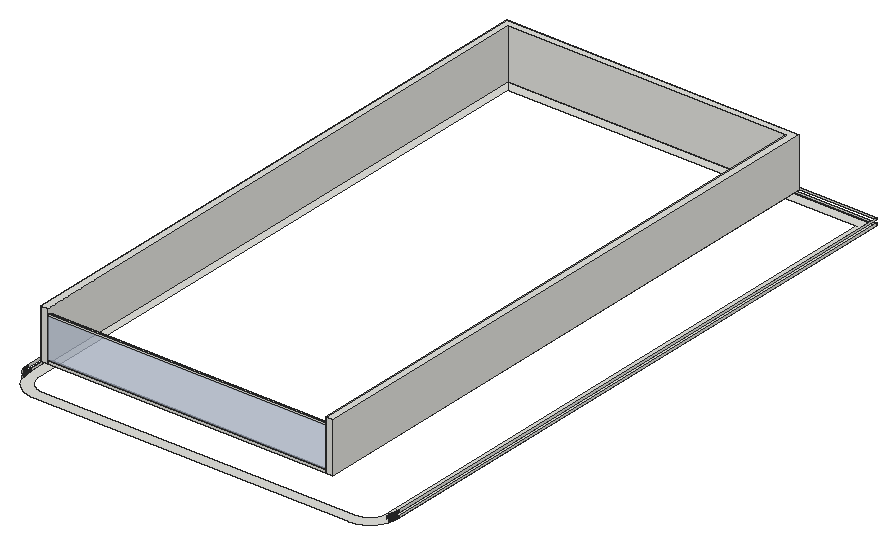
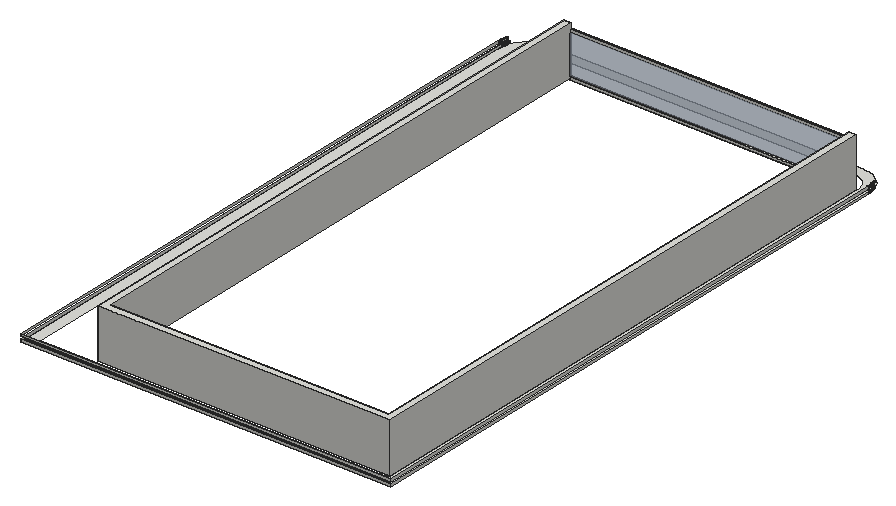
# SketchUp Ruby script. Lengths in inches.
U = 1.inch
M = Sketchup.active_model
def pt(a) = Geom::Point3d.new(a.map { |v| v * U })
def face(e, loops, mat)
  f = e.add_face(loops[0].map { |a| pt(a) })
  loops[1..].each { |l| e.add_face(l.map { |a| pt(a) }).erase! }
  f.material = f.back_material = mat if mat
  f
end
# faces: each face lists its corners as indices into pts; further lists are holes
def faces(e, pts, list, mat = nil) = list.each { |f| face(e, (f[0].is_a?(Array) ? f : [f]).map { |l| l.map { |i| pts[i] } }, mat) }
# xy, xz, yz: faces in a plane at the given z, y or x. An outline is a flat list of corners, or four numbers for a rectangle; further outlines are holes
def ring(l) = l.size == 4 ? [[l[0], l[1]], [l[2], l[1]], [l[2], l[3]], [l[0], l[3]]] : l.each_slice(2).to_a
def flat(e, list, mat, &to3) = list.each { |f| face(e, (f[0].is_a?(Array) ? f : [f]).map { |l| ring(l).map { |u, v| to3.(u, v) } }, mat) }
def xy(e, z, list, mat = nil) = flat(e, list, mat) { |x, y| [x, y, z] }
def xz(e, y, list, mat = nil) = flat(e, list, mat) { |x, z| [x, y, z] }
def yz(e, x, list, mat = nil) = flat(e, list, mat) { |y, z| [x, y, z] }
def lines(e, pts, list) = list.each { |a, b| e.add_line(pt(pts[a]), pt(pts[b])) }
# prism: a flat outline (further loops are holes) pulled along v
def prism(e, loops, v, mat = nil)
  f = face(e, loops, mat); d = Geom::Vector3d.new(v.map { |x| x * U })
  f.pushpull(f.normal.samedirection?(d) ? d.length : -d.length)
end
def box(e, o, s, mat = nil) = prism(e, [[o, [o[0] + s[0], o[1], o[2]], [o[0] + s[0], o[1] + s[1], o[2]], [o[0], o[1] + s[1], o[2]]]], [0, 0, s[2]], mat)
def at(x, y, z, deg = 0) = Geom::Transformation.translation(pt([x, y, z])) * Geom::Transformation.rotation(ORIGIN, Z_AXIS, deg.degrees)
def axes(o, x, y, z) = Geom::Transformation.new([*x, 0, *y, 0, *z, 0, *pt(o).to_a, 1])
def part(name) = M.definitions.add(name)
# library, detail: a bought-in or finely detailed component or shape, given as its bounding box
def library(name, o, s) = part(name).tap { |d| box(d.entities, o, s) }
def detail(e, o, s) = box(e.add_group.entities, o, s)
def put(e, d, t, mat = nil) = e.add_instance(d, t).tap { |i| i.material = mat if mat }
def group(e, t, mat = nil) = e.add_group.tap { |g| g.transformation = t; g.material = mat if mat }.entities
root = M.entities
M.materials.add("[Translucent Glass Blue]").color = [196, 207, 226]
M.materials["[Translucent Glass Blue]"].alpha = 0.5
xy(root,392.81,[[[26,144,290.77,144,291.08,144.01,291.4,144.02,291.71,144.03,292.02,144.05,292.34,144.08,292.65,144.1,292.96,144.13,293.27,144.17,293.59,144.21,293.9,144.25,294.83,144.4,295.14,144.46,295.44,144.53,295.75,144.59,296.06,144.67,296.36,144.74,296.67,144.82,296.97,144.9,297.57,145.08,298.17,145.28,298.46,145.38,298.76,145.49,299.05,145.6,299.35,145.71,299.93,145.95,300.22,146.08,300.5,146.21,300.79,146.34,301.63,146.76,301.91,146.91,302.18,147.0625,302.45,147.22,302.72,147.375,302.99,147.54,303.26,147.7,303.52,147.875,303.79,148.05,304.05,148.22,304.3,148.4,304.56,148.59,304.8125,148.77,305.3125,149.15,305.56,149.35,306.04,149.75,306.28,149.96,306.97,150.59,307.2,150.8125,307.42,151.03,307.64,151.26,307.86,151.48,308.08,151.71,308.29,151.94,308.5,152.18,308.7,152.42,308.91,152.66,309.1,152.9,309.3,153.14,309.68,153.64,309.87,153.9,310.05,154.15,310.41,154.67,310.58,154.93,310.75,155.2,310.92,155.46,311.24,156,311.39,156.28,311.55,156.55,311.69,156.83,311.84,157.11,312.12,157.67,312.25,157.95,312.38,158.24,312.5,158.53,312.625,158.82,312.74,159.11,312.86,159.4,312.97,159.7,313.08,159.99,313.28,160.59,313.375,160.89,313.47,161.1875,313.55,161.49,313.64,161.79,313.71,162.09,313.79,162.4,313.86,162.71,313.93,163.01,314.05,163.63,314.11,163.9375,314.16,164.25,314.21,164.56,314.29,165.18,314.32,165.49,314.35,165.81,314.38,166.12,314.4,166.43,314.42,166.75,314.43,167.06,314.45,167.375,314.45,672,2,672,2,168,2.21,164.87,2.82,161.79,3.83,158.82,5.22,156,6.96,153.39,9.03,151.03,11.39,148.96,14,147.22,16.82,145.83,19.79,144.82,22.87,144.21],[26,153,24.04,153.13,22.12,153.51,20.26,154.14,18.5,155.01,16.87,156.1,15.39,157.4,14.1,158.87,13.01,160.5,12.14,162.26,11.51,164.12,11.13,166.04,11,168,11,663,305,663,305,164.34,304.99,164.31,304.84,163.74,304.78,163.55,304.72,163.37,304.66,163.18,304.59,162.99,304.53,162.81,304.39,162.44,304.3125,162.26,304.24,162.08,304.08,161.72,303.99,161.54,303.91,161.37,303.82,161.19,303.73,161.02,303.64,160.84,303.24,160.16,303.14,160,303.03,159.83,302.93,159.67,302.82,159.51,302.7,159.34,302.59,159.19,302.35,158.87,302.23,158.72,302.11,158.5625,301.99,158.41,301.73,158.11,301.6,157.97,301.47,157.82,301.33,157.68,301.2,157.54,300.78,157.12,300.64,156.99,300.49,156.85,300.34,156.72,300.2,156.6,300.04,156.47,299.89,156.34,299.74,156.22,299.58,156.1,299.43,155.98,299.27,155.87,299.11,155.75,298.79,155.53,298.62,155.42,298.46,155.32,298.29,155.21,297.78,154.91,297.61,154.82,297.4375,154.73,297.26,154.64,297.09,154.55,296.91,154.46,296.55,154.3,296.375,154.22,296.19,154.14,295.65,153.93,295.46,153.86,295.27,153.8,295.09,153.74,294.71,153.62,294.53,153.57,294.34,153.51,294.15,153.46,293.96,153.42,293.76,153.37,293.38,153.29,293.1875,153.25,292.99,153.22,292.8,153.1875,292.61,153.16,292.41,153.13,292.22,153.11,292.02,153.08,291.83,153.06,291.63,153.05,291.43,153.03,291.24,153.02,291.04,153.01,290.85,153.01,290.65,153]]])
xy(root,398.81,[[5,177.03,11,177.03,11,663,251.45,663,251.45,669,5,669],[245.45,177.03,251.45,663]])
xy(root,440.81,[[5,177.03,11,177.03,11,663,245.45,663,245.45,177.03,251.45,177.03,251.45,669,5,669]])
xz(root,177.03,[[5,398.81,11,440.81],[245.45,398.81,251.45,440.81]])
xz(root,663,[[11,398.81,245.45,440.81]])
xz(root,669,[[5,398.81,251.45,440.81]])
xz(root,670,[[4,394.81,312.45,396.81]])
xz(root,672,[[2,392.81,314.45,394.81],[2,396.81,314.45,398.81]])
yz(root,2,[[167.68,392.81,168,394.81],[168,392.81,672,394.81],[167.68,396.81,168,398.81],[168,396.81,672,398.81]])
yz(root,4,[[167.71,394.81,168.01,396.81],[168.01,394.81,670,396.81]])
yz(root,5,[[177.03,398.81,669,440.81]])
yz(root,11,[[177.03,398.81,663,440.81]])
yz(root,245.45,[[177.03,398.81,663,440.81]])
yz(root,251.45,[[177.03,398.81,669,440.81]])
yz(root,312.45,[[167.42,394.81,167.71,396.81],[167.71,394.81,168.01,396.81],[168.01,394.81,670,396.81]])
yz(root,314.45,[[167.37,392.81,167.68,394.81],[167.68,392.81,168,394.81],[168,392.81,672,394.81],[167.37,396.81,167.68,398.81],[167.68,396.81,168,398.81],
  [168,396.81,672,398.81]])
p = [[3.38,159.99,392.81],[3.49,159.69,392.81],[3.49,159.69,394.81],[3.38,159.99,394.81],[312.97,159.69,392.81],[313.07,159.99,392.81],
  [313.07,159.99,394.81],[312.97,159.69,394.81],[3.28,160.28,392.81],[3.28,160.28,394.81],[313.18,160.28,392.81],[313.18,160.28,394.81],
  [3.18,160.58,392.81],[3.18,160.58,394.81],[313.28,160.58,392.81],[313.28,160.58,394.81],[3.08,160.88,392.81],[3.08,160.88,394.81],
  [313.37,160.88,392.81],[313.37,160.88,394.81],[2.99,161.18,392.81],[2.99,161.18,394.81],[313.46,161.18,392.81],[313.46,161.18,394.81],
  [2.9,161.48,392.81],[2.9,161.48,394.81],[313.55,161.48,392.81],[313.55,161.48,394.81],[2.82,161.79,392.81],[2.82,161.79,394.81],
  [313.63,161.79,392.81],[313.63,161.79,394.81],[2.74,162.09,392.81],[2.74,162.09,394.81],[313.71,162.09,392.81],[313.71,162.09,394.81],
  [2.66,162.4,392.81],[2.66,162.4,394.81],[313.79,162.4,392.81],[313.79,162.4,394.81],[2.59,162.7,392.81],[2.59,162.7,394.81],
  [313.86,162.7,392.81],[313.86,162.7,394.81],[2.53,163.01,392.81],[2.53,163.01,394.81],[313.93,163.01,392.81],[313.93,163.01,394.81],
  [2.46,163.32,392.81],[2.46,163.32,394.81],[313.99,163.32,392.81],[313.99,163.32,394.81],[2.4,163.625,392.81],[2.4,163.625,394.81],
  [314.05,163.625,392.81],[314.05,163.625,394.81],[2.35,163.93,392.81],[2.35,163.93,394.81],[314.11,163.93,392.81],[314.11,163.93,394.81],
  [2.3,164.24,392.81],[2.3,164.24,394.81],[314.16,164.24,392.81],[314.16,164.24,394.81],[2.25,164.55,392.81],[2.25,164.55,394.81],
  [314.2,164.55,392.81],[314.2,164.55,394.81],[2.21,164.87,392.81],[2.21,164.87,394.81],[314.25,164.87,392.81],[314.25,164.87,394.81],
  [2.17,165.18,392.81],[2.17,165.18,394.81],[314.29,165.18,392.81],[314.29,165.18,394.81],[2.13,165.49,392.81],[2.13,165.49,394.81],
  [314.32,165.49,392.81],[314.32,165.49,394.81],[2.1,165.8,392.81],[2.1,165.8,394.81],[314.35,165.8,392.81],[314.35,165.8,394.81],
  [2.07,166.12,392.81],[2.07,166.12,394.81],[314.38,166.12,392.81],[314.38,166.12,394.81],[2.05,166.43,392.81],[2.05,166.43,394.81],
  [314.4,166.43,392.81],[314.4,166.43,394.81],[2.03,166.74,392.81],[2.03,166.74,394.81],[314.42,166.74,392.81],[314.42,166.74,394.81],
  [2.02,167.06,392.81],[2.02,167.06,394.81],[314.43,167.06,392.81],[314.43,167.06,394.81],[2.01,167.37,392.81],[2.01,167.37,394.81],
  [314.45,167.37,392.81],[314.45,167.37,394.81],[2,167.68,392.81],[2,167.68,394.81],[5.46,160.12,394.81],[5.57,159.85,394.81],
  [5.57,159.85,396.81],[5.46,160.12,396.81],[310.89,159.85,394.81],[310.99,160.12,394.81],[310.99,160.12,396.81],[310.89,159.85,396.81],
  [5.36,160.39,394.81],[5.36,160.39,396.81],[311.09,160.39,394.81],[311.09,160.39,396.81],[5.26,160.66,394.81],[5.26,160.66,396.81],
  [311.19,160.66,394.81],[311.19,160.66,396.81],[5.17,160.93,394.81],[5.17,160.93,396.81],[311.28,160.93,394.81],[311.28,160.93,396.81],
  [5.08,161.2,394.81],[5.08,161.2,396.81],[311.375,161.2,394.81],[311.375,161.2,396.81],[4.99,161.48,394.81],[4.99,161.48,396.81],
  [311.46,161.48,394.81],[311.46,161.48,396.81],[4.91,161.75,394.81],[4.91,161.75,396.81],[311.55,161.75,394.81],[311.55,161.75,396.81],
  [4.83,162.03,394.81],[4.83,162.03,396.81],[311.625,162.03,394.81],[311.625,162.03,396.81],[4.75,162.31,394.81],[4.75,162.31,396.81],
  [311.7,162.31,394.81],[311.7,162.31,396.81],[4.68,162.58,394.81],[4.68,162.58,396.81],[311.78,162.58,394.81],[311.78,162.58,396.81],
  [4.61,162.86,394.81],[4.61,162.86,396.81],[311.84,162.86,394.81],[311.84,162.86,396.81],[4.54,163.14,394.81],[4.54,163.14,396.81],
  [311.91,163.14,394.81],[311.91,163.14,396.81],[4.48,163.43,394.81],[4.48,163.43,396.81],[311.97,163.43,394.81],[311.97,163.43,396.81],
  [4.42,163.71,394.81],[4.42,163.71,396.81],[312.03,163.71,394.81],[312.03,163.71,396.81],[4.37,163.99,394.81],[4.37,163.99,396.81],
  [312.08,163.99,394.81],[312.08,163.99,396.81],[4.32,164.27,394.81],[4.32,164.27,396.81],[312.14,164.27,394.81],[312.14,164.27,396.81],
  [4.27,164.56,394.81],[4.27,164.56,396.81],[312.18,164.56,394.81],[312.18,164.56,396.81],[4.23,164.84,394.81],[4.23,164.84,396.81],
  [312.23,164.84,394.81],[312.23,164.84,396.81],[4.1875,165.13,394.81],[4.1875,165.13,396.81],[312.26,165.13,394.81],[312.26,165.13,396.81],
  [4.15,165.41,394.81],[4.15,165.41,396.81],[312.3,165.41,394.81],[312.3,165.41,396.81],[4.12,165.7,394.81],[4.12,165.7,396.81],
  [312.33,165.7,394.81],[312.33,165.7,396.81],[4.09,165.99,394.81],[4.09,165.99,396.81],[312.36,165.99,394.81],[312.36,165.99,396.81],
  [4.07,166.27,394.81],[4.07,166.27,396.81],[312.39,166.27,394.81],[312.39,166.27,396.81],[4.05,166.56,394.81],[4.05,166.56,396.81],
  [312.41,166.56,394.81],[312.41,166.56,396.81],[4.03,166.85,394.81],[4.03,166.85,396.81],[312.42,166.85,394.81],[312.42,166.85,396.81],
  [4.02,167.14,394.81],[4.02,167.14,396.81],[312.4375,167.14,394.81],[312.4375,167.14,396.81],[4.01,167.42,394.81],[4.01,167.42,396.81],
  [312.45,167.42,394.81],[312.45,167.42,396.81],[4,167.71,394.81],[4,167.71,396.81],[3.38,159.99,396.81],[3.49,159.69,396.81],
  [3.49,159.69,398.81],[3.38,159.99,398.81],[312.97,159.69,396.81],[313.07,159.99,396.81],[313.07,159.99,398.81],[312.97,159.69,398.81],
  [3.28,160.28,396.81],[3.28,160.28,398.81],[313.18,160.28,396.81],[313.18,160.28,398.81],[3.18,160.58,396.81],[3.18,160.58,398.81],
  [313.28,160.58,396.81],[313.28,160.58,398.81],[3.08,160.88,396.81],[3.08,160.88,398.81],[313.37,160.88,396.81],[313.37,160.88,398.81],
  [2.99,161.18,396.81],[2.99,161.18,398.81],[313.46,161.18,396.81],[313.46,161.18,398.81],[2.9,161.48,396.81],[2.9,161.48,398.81],
  [313.55,161.48,396.81],[313.55,161.48,398.81],[2.82,161.79,396.81],[2.82,161.79,398.81],[313.63,161.79,396.81],[313.63,161.79,398.81],
  [2.74,162.09,396.81],[2.74,162.09,398.81],[313.71,162.09,396.81],[313.71,162.09,398.81],[2.66,162.4,396.81],[2.66,162.4,398.81],
  [313.79,162.4,396.81],[313.79,162.4,398.81],[2.59,162.7,396.81],[2.59,162.7,398.81],[313.86,162.7,396.81],[313.86,162.7,398.81],
  [2.53,163.01,396.81],[2.53,163.01,398.81],[313.93,163.01,396.81],[313.93,163.01,398.81],[2.46,163.32,396.81],[2.46,163.32,398.81],
  [313.99,163.32,396.81],[313.99,163.32,398.81],[2.4,163.625,396.81],[2.4,163.625,398.81],[314.05,163.625,396.81],[314.05,163.625,398.81],
  [2.35,163.93,396.81],[2.35,163.93,398.81],[314.11,163.93,396.81],[314.11,163.93,398.81],[2.3,164.24,396.81],[2.3,164.24,398.81],
  [314.16,164.24,396.81],[314.16,164.24,398.81],[2.25,164.55,396.81],[2.25,164.55,398.81],[314.2,164.55,396.81],[314.2,164.55,398.81],
  [2.21,164.87,396.81],[2.21,164.87,398.81],[314.25,164.87,396.81],[314.25,164.87,398.81],[2.17,165.18,396.81],[2.17,165.18,398.81],
  [314.29,165.18,396.81],[314.29,165.18,398.81],[2.13,165.49,396.81],[2.13,165.49,398.81],[314.32,165.49,396.81],[314.32,165.49,398.81],
  [2.1,165.8,396.81],[2.1,165.8,398.81],[314.35,165.8,396.81],[314.35,165.8,398.81],[2.07,166.12,396.81],[2.07,166.12,398.81],
  [314.38,166.12,396.81],[314.38,166.12,398.81],[2.05,166.43,396.81],[2.05,166.43,398.81],[314.4,166.43,396.81],[314.4,166.43,398.81],
  [2.03,166.74,396.81],[2.03,166.74,398.81],[314.42,166.74,396.81],[314.42,166.74,398.81],[2.02,167.06,396.81],[2.02,167.06,398.81],
  [314.43,167.06,396.81],[314.43,167.06,398.81],[2.01,167.37,396.81],[2.01,167.37,398.81],[314.45,167.37,396.81],[314.45,167.37,398.81],
  [2,167.68,396.81],[2,167.68,398.81],[305.45,663,392.81],[305,663,392.81],[11,663,398.81],[11,663,392.81],
  [312.45,168.01,396.81],[312.45,168.01,398.81],[4,670,396.81],[4,670,398.81],[4,168.01,396.81],[4,168.01,398.81]]
faces(root,p,[[0,1,2,3],[4,5,6,7],[8,0,3,9],[5,10,11,6],[12,8,9,13],[10,14,15,11],[16,12,13,17],[14,18,19,15],
  [20,16,17,21],[18,22,23,19],[24,20,21,25],[22,26,27,23],[28,24,25,29],[26,30,31,27],[32,28,29,33],[30,34,35,31],
  [36,32,33,37],[34,38,39,35],[40,36,37,41],[38,42,43,39],[44,40,41,45],[42,46,47,43],[48,44,45,49],[46,50,51,47],
  [52,48,49,53],[50,54,55,51],[56,52,53,57],[54,58,59,55],[60,56,57,61],[58,62,63,59],[64,60,61,65],[62,66,67,63],
  [68,64,65,69],[66,70,71,67],[72,68,69,73],[70,74,75,71],[76,72,73,77],[74,78,79,75],[80,76,77,81],[78,82,83,79],
  [84,80,81,85],[82,86,87,83],[88,84,85,89],[86,90,91,87],[92,88,89,93],[90,94,95,91],[96,92,93,97],[94,98,99,95],
  [100,96,97,101],[98,102,103,99],[104,100,101,105],[106,107,108,109],[110,111,112,113],[114,106,109,115],[111,116,117,112],[118,114,115,119],
  [116,120,121,117],[122,118,119,123],[120,124,125,121],[126,122,123,127],[124,128,129,125],[130,126,127,131],[128,132,133,129],[134,130,131,135],
  [132,136,137,133],[138,134,135,139],[136,140,141,137],[142,138,139,143],[140,144,145,141],[146,142,143,147],[144,148,149,145],[150,146,147,151],
  [148,152,153,149],[154,150,151,155],[152,156,157,153],[158,154,155,159],[156,160,161,157],[162,158,159,163],[160,164,165,161],[166,162,163,167],
  [164,168,169,165],[170,166,167,171],[168,172,173,169],[174,170,171,175],[172,176,177,173],[178,174,175,179],[176,180,181,177],[182,178,179,183],
  [180,184,185,181],[186,182,183,187],[184,188,189,185],[190,186,187,191],[188,192,193,189],[194,190,191,195],[192,196,197,193],[198,194,195,199],
  [196,200,201,197],[202,198,199,203],[200,204,205,201],[206,202,203,207],[204,208,209,205],[210,206,207,211],[208,212,213,209],[214,210,211,215],
  [212,216,217,213],[218,214,215,219],[220,221,222,223],[224,225,226,227],[228,220,223,229],[225,230,231,226],[232,228,229,233],[230,234,235,231],
  [236,232,233,237],[234,238,239,235],[240,236,237,241],[238,242,243,239],[244,240,241,245],[242,246,247,243],[248,244,245,249],[246,250,251,247],
  [252,248,249,253],[250,254,255,251],[256,252,253,257],[254,258,259,255],[260,256,257,261],[258,262,263,259],[264,260,261,265],[262,266,267,263],
  [268,264,265,269],[266,270,271,267],[272,268,269,273],[270,274,275,271],[276,272,273,277],[274,278,279,275],[280,276,277,281],[278,282,283,279],
  [284,280,281,285],[282,286,287,283],[288,284,285,289],[286,290,291,287],[292,288,289,293],[290,294,295,291],[296,292,293,297],[294,298,299,295],
  [300,296,297,301],[298,302,303,299],[304,300,301,305],[302,306,307,303],[308,304,305,309],[306,310,311,307],[312,308,309,313],[310,314,315,311],
  [316,312,313,317],[314,318,319,315],[320,316,317,321],[318,322,323,319],[324,320,321,325]])
lines(root,p,[[326,327],[328,329],[330,331],[332,333],[334,335]])
g1 = group(root,at(11,177.03,398.81))
box(g1,[0,0,0],[234.45,2,2])
box(g1,[0,0,36],[234.45,2,2])
g2 = group(g1,at(0,0.75,2),"[Translucent Glass Blue]")
box(g2,[0,0,0],[234.45,0.5,34])
